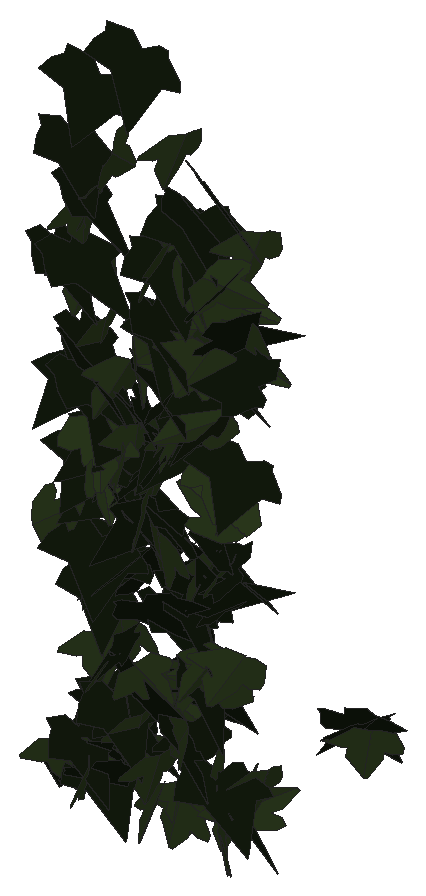
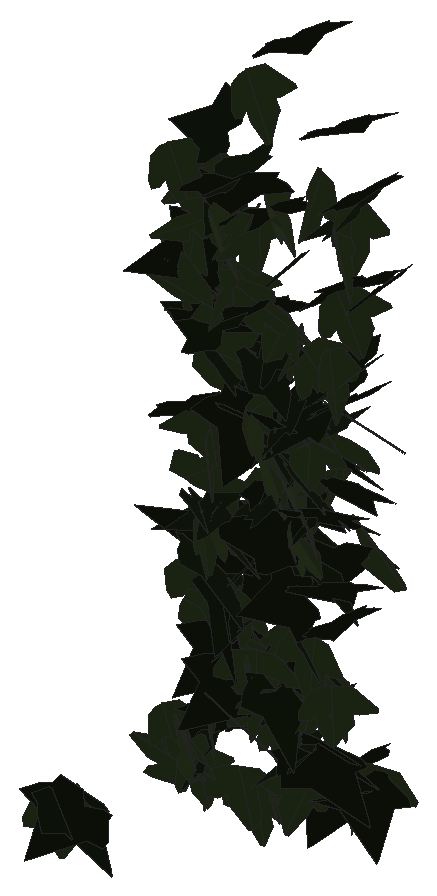
# SketchUp Ruby script. Lengths in inches.
U = 1.inch
M = Sketchup.active_model
def pt(a) = Geom::Point3d.new(a.map { |v| v * U })
def face(e, loops, mat)
  f = e.add_face(loops[0].map { |a| pt(a) })
  loops[1..].each { |l| e.add_face(l.map { |a| pt(a) }).erase! }
  f.material = f.back_material = mat if mat
  f
end
# faces: each face lists its corners as indices into pts; further lists are holes
def faces(e, pts, list, mat = nil) = list.each { |f| face(e, (f[0].is_a?(Array) ? f : [f]).map { |l| l.map { |i| pts[i] } }, mat) }
# xy, xz, yz: faces in a plane at the given z, y or x. An outline is a flat list of corners, or four numbers for a rectangle; further outlines are holes
def ring(l) = l.size == 4 ? [[l[0], l[1]], [l[2], l[1]], [l[2], l[3]], [l[0], l[3]]] : l.each_slice(2).to_a
def flat(e, list, mat, &to3) = list.each { |f| face(e, (f[0].is_a?(Array) ? f : [f]).map { |l| ring(l).map { |u, v| to3.(u, v) } }, mat) }
def xy(e, z, list, mat = nil) = flat(e, list, mat) { |x, y| [x, y, z] }
def xz(e, y, list, mat = nil) = flat(e, list, mat) { |x, z| [x, y, z] }
def yz(e, x, list, mat = nil) = flat(e, list, mat) { |y, z| [x, y, z] }
def lines(e, pts, list) = list.each { |a, b| e.add_line(pt(pts[a]), pt(pts[b])) }
# prism: a flat outline (further loops are holes) pulled along v
def prism(e, loops, v, mat = nil)
  f = face(e, loops, mat); d = Geom::Vector3d.new(v.map { |x| x * U })
  f.pushpull(f.normal.samedirection?(d) ? d.length : -d.length)
end
def box(e, o, s, mat = nil) = prism(e, [[o, [o[0] + s[0], o[1], o[2]], [o[0] + s[0], o[1] + s[1], o[2]], [o[0], o[1] + s[1], o[2]]]], [0, 0, s[2]], mat)
def at(x, y, z, deg = 0) = Geom::Transformation.translation(pt([x, y, z])) * Geom::Transformation.rotation(ORIGIN, Z_AXIS, deg.degrees)
def axes(o, x, y, z) = Geom::Transformation.new([*x, 0, *y, 0, *z, 0, *pt(o).to_a, 1])
def part(name) = M.definitions.add(name)
# library, detail: a bought-in or finely detailed component or shape, given as its bounding box
def library(name, o, s) = part(name).tap { |d| box(d.entities, o, s) }
def detail(e, o, s) = box(e.add_group.entities, o, s)
def put(e, d, t, mat = nil) = e.add_instance(d, t).tap { |i| i.material = mat if mat }
def group(e, t, mat = nil) = e.add_group.tap { |g| g.transformation = t; g.material = mat if mat }.entities
root = M.entities
M.materials.add("1026 AP 7946 SUNNY SIDE UP").color = [254, 231, 186]
M.materials.add("efeu1").color = [18, 25, 13]
M.materials.add("efeu2").color = [43, 57, 29]
c1 = part("ivyleaf_10")
p = [[0,0.5,-0.03],[-0.0625,2.02,-0.43],[-0.19,2.01,-0.46],[-0.54,1.05,-0.29],[-0.52,0.625,-0.18],[-0.83,0.76,-0.28],
  [-1.16,0.64,-0.33],[-1.15,0.33,-0.24],[-0.77,-0.39,0.02],[-0.3,-0.51,0.16],[0.04,-0.48,0.23],[-0.02,2.01,-0.4375],
  [-0.06,2.01,-0.43],[0.04,-0.49,0.23],[0.67,-0.49,0.14],[1.38,0.36,-0.2],[1.375,0.51,-0.24],[0.81,0.65,-0.19],
  [0.62,0.59,-0.15],[0.6,1.09,-0.28],[0.5,1.23,-0.31]]
faces(c1.entities,p,[[0,1,2,3,4,5,6,7,8,9,10],[11,12,0,13,14,15,16,17,18,19,20]],"efeu2")
c2 = part("ivyleaf_9")
p = [[1.54,2.16,1.25],[1.36,2.04,1.19],[-0.21,0.99,0.68],[-0.71,1.11,0.82],[-0.85,0.86,0.67],[-0.8,0.17,0.21],
  [-0.9,-0.01,0.1],[-0.67,-0.16,-0.02],[-0.08,-0.08,-0.05],[-0.03,-0.6,-0.4],[0.65,-0.88,-0.66],[0.83,-0.6,-0.49],
  [1.29,-0.42,-0.43],[1.8125,-0.07,-0.26],[1.21,0.44,0.15]]
faces(c2.entities,p,[[0,1,2,3,4,5,6,7,8,9,10,11,12,13,14]],"efeu1")
put(root,c1,axes([128.77,212.34,283.15],[0.31487,-0.18449,-0.22671],[0.28999,-0.12137,0.27832],[-0.34447,-0.27081,0.02707]),"1026 AP 7946 SUNNY SIDE UP")
put(root,c2,axes([128.875,212.4,287.29],[0.16277,-0.31766,-0.09668],[-0.03791,0.08894,-0.34364],[0.51865,0.10619,0.00522]),"1026 AP 7946 SUNNY SIDE UP")
put(root,c2,axes([129.22,212.62,285.39],[-0.49049,-0.04517,-0.10193],[0.16934,-0.09172,-0.30799],[0.02108,-0.31405,0.10257]),"1026 AP 7946 SUNNY SIDE UP")
put(root,c2,axes([128.96,212.68,288.75],[-0.00054,-0.35085,-0.02221],[0.01961,0.01954,-0.3611],[0.55219,-0.00104,0.0128]),"1026 AP 7946 SUNNY SIDE UP")
put(root,c2,axes([129.28,212.29,279.97],[0.19093,0.26653,-0.14134],[-0.09154,-0.12591,-0.30246],[-0.4635,0.13466,0.00151]),"1026 AP 7946 SUNNY SIDE UP")
put(root,c1,axes([129.2,212.18,280],[-0.40377,-0.18367,-0.07564],[0.11643,0.02048,-0.32404],[0.28776,-0.266,0.02498]),"1026 AP 7946 SUNNY SIDE UP")
put(root,c1,axes([129.27,212.73,287.93],[0.13295,-0.33199,-0.07426],[-0.00651,0.07133,-0.35224],[0.53352,0.0836,0.01421]),"1026 AP 7946 SUNNY SIDE UP")
put(root,c1,axes([129.3,212.62,286.95],[-0.20815,-0.31172,0.08991],[0.00262,-0.09684,-0.34724],[0.50974,-0.12679,0.0385]),"1026 AP 7946 SUNNY SIDE UP")
put(root,c2,axes([129.25,212.82,289.65],[-0.24116,-0.30442,0.09077],[0.00826,-0.10219,-0.34812],[0.49901,-0.14543,0.04962]),"1026 AP 7946 SUNNY SIDE UP")
put(root,c1,axes([129.36,212.79,281.35],[-0.30602,-0.25261,0.0146],[0.0642,-0.05076,-0.32229],[0.39275,-0.18853,0.06405]),"1026 AP 7946 SUNNY SIDE UP")
put(root,c1,axes([129.37,212.35,288.04],[-0.0998,-0.33764,-0.07705],[0.04363,0.06887,-0.35322],[0.54138,-0.06779,0.01426]),"1026 AP 7946 SUNNY SIDE UP")
put(root,c1,axes([129.4,212.71,286.11],[-0.02529,-0.33428,-0.08226],[0.01042,0.07772,-0.3443],[0.53962,-0.01717,0.00279]),"1026 AP 7946 SUNNY SIDE UP")
put(root,c2,axes([129.13,212.65,286.02],[0.19765,-0.30445,-0.09302],[-0.01495,0.09161,-0.33779],[0.49833,0.1235,0.02676]),"1026 AP 7946 SUNNY SIDE UP")
put(root,c2,axes([129.6,212.85,280.47],[0.14491,0.11175,-0.28967],[-0.24026,-0.23728,-0.14979],[-0.41172,0.1778,-0.01454]),"1026 AP 7946 SUNNY SIDE UP")
put(root,c2,axes([129.16,212.41,287.3],[0.12708,-0.29012,-0.17529],[0.07618,0.1816,-0.29711],[0.52202,0.04413,0.08603]),"1026 AP 7946 SUNNY SIDE UP")
put(root,c2,axes([129.54,212.59,284.34],[-0.46172,-0.14613,-0.05063],[0.11028,-0.0344,-0.33213],[0.21543,-0.29559,0.06151]),"1026 AP 7946 SUNNY SIDE UP")
put(root,c2,axes([129.24,212.43,288.28],[0.27121,-0.30689,-0.07246],[-0.0126,0.07392,-0.36103],[0.49431,0.17027,0.03055]),"1026 AP 7946 SUNNY SIDE UP")
put(root,c2,axes([129.36,212.3,280.26],[0.04395,-0.30745,-0.10444],[-0.01885,0.09895,-0.31744],[0.50783,0.03028,-0.00274]),"1026 AP 7946 SUNNY SIDE UP")
put(root,c1,axes([129.55,212.77,288.64],[-0.00548,-0.23836,-0.29542],[0.05999,0.28368,-0.2429],[0.58161,-0.03151,0.02227]),"1026 AP 7946 SUNNY SIDE UP")
put(root,c2,axes([129.4375,212.67,282.38],[-0.09606,-0.32529,0.02138],[-0.00287,-0.02265,-0.3411],[0.51272,-0.06107,0.0021]),"1026 AP 7946 SUNNY SIDE UP")
put(root,c2,axes([129.77,212.75,280.62],[-0.50354,0.00349,-0.01504],[0.02207,-0.04213,-0.32733],[-0.00845,-0.31779,0.04134]),"1026 AP 7946 SUNNY SIDE UP")
put(root,c2,axes([129.29,212.41,285.57],[0.19261,-0.28911,-0.16675],[0.0311,0.17697,-0.31237],[0.5188,0.09673,0.08063]),"1026 AP 7946 SUNNY SIDE UP")
put(root,c1,axes([129.61,212.09,279.8125],[0.10943,-0.27423,-0.15568],[-0.01177,0.15172,-0.28929],[0.49101,0.06475,0.02776]),"1026 AP 7946 SUNNY SIDE UP")
put(root,c2,axes([129.58,212.78,282.88],[-0.32897,-0.25226,0.02968],[0.03288,-0.05614,-0.33372],[0.39814,-0.2038,0.05209]),"1026 AP 7946 SUNNY SIDE UP")
put(root,c2,axes([129.31,212.26,285.95],[0.32591,-0.26952,0.0464],[0.01664,-0.05049,-0.34982],[0.42975,0.20635,-0.02164]),"1026 AP 7946 SUNNY SIDE UP")
put(root,c1,axes([129.65,212.46,281.25],[0.11967,-0.31363,-0.0036],[-0.01012,0.0002,-0.33242],[0.49306,0.07612,-0.00595]),"1026 AP 7946 SUNNY SIDE UP")
put(root,c2,axes([129.8,212.78,283.88],[-0.46379,-0.1306,0.08783],[-0.06846,-0.10776,-0.32304],[0.23616,-0.28772,0.07885]),"1026 AP 7946 SUNNY SIDE UP")
put(root,c1,axes([129.8,212.68,281.86],[-0.48011,0.0946,0.04933],[-0.08062,-0.00584,-0.32866],[-0.14549,-0.30893,0.01934]),"1026 AP 7946 SUNNY SIDE UP")
put(root,c2,axes([129.65,212.21,279.81],[0.32277,0.23557,-0.0003],[0.02221,-0.01446,-0.32131],[-0.36975,0.20477,-0.01956]),"1026 AP 7946 SUNNY SIDE UP")
put(root,c2,axes([129.91,212.51,284.73],[-0.52122,-0.00918,-0.03163],[0.05013,-0.06745,-0.33475],[0.0043,-0.32599,0.06817]),"1026 AP 7946 SUNNY SIDE UP")
put(root,c2,axes([129.55,212.52,279.73],[-0.06473,-0.30275,-0.08361],[0.09228,0.07124,-0.3106],[0.48343,-0.05413,0.04809]),"1026 AP 7946 SUNNY SIDE UP")
put(root,c1,axes([129.86,212.67,284.86],[-0.51512,0.04532,0.04355],[-0.07068,-0.01925,-0.33984],[-0.06667,-0.32972,0.02385]),"1026 AP 7946 SUNNY SIDE UP")
put(root,c2,axes([129.7,212.31,283.19],[-0.34121,-0.2423,-0.11903],[0.14727,0.06902,-0.33389],[0.39458,-0.23528,0.02168]),"1026 AP 7946 SUNNY SIDE UP")
put(root,c1,axes([129.63,212.31,284.76],[0.53185,-0.01594,0.1042],[0.15511,-0.04395,-0.34694],[0.04366,0.35032,-0.0367]),"1026 AP 7946 SUNNY SIDE UP")
put(root,c1,axes([129.74,212.3,284.23],[0.09294,0.32094,-0.02856],[0.00039,-0.03008,-0.33632],[-0.50679,0.05883,-0.0055]),"1026 AP 7946 SUNNY SIDE UP")
put(root,c1,axes([129.77,212.78,279.95],[0.23329,0.24155,0.15104],[-0.03258,0.17303,-0.27365],[-0.44198,0.11474,0.09989]),"1026 AP 7946 SUNNY SIDE UP")
put(root,c2,axes([129.74,212.53,284.91],[-0.16662,-0.25075,0.2084],[0.03989,-0.22019,-0.2669],[0.50642,-0.06516,0.08959]),"1026 AP 7946 SUNNY SIDE UP")
put(root,c2,axes([130.01,212.77,284.41],[-0.44334,0.11575,-0.13747],[0.16419,-0.09502,-0.31123],[-0.225,-0.29741,0.04375]),"1026 AP 7946 SUNNY SIDE UP")
put(root,c1,axes([130.01,212.36,285.8],[-0.09987,-0.30957,0.16238],[-0.00305,-0.16169,-0.32529],[0.54749,-0.05737,0.02781]),"1026 AP 7946 SUNNY SIDE UP")
put(root,c2,axes([129.76,212.55,285.33],[0.45438,-0.12423,-0.13502],[-0.16783,0.08034,-0.32217],[0.22805,0.30667,0.03192]),"1026 AP 7946 SUNNY SIDE UP")
put(root,c1,axes([129.95,212.69,283.9],[0.25028,-0.2959,0.01977],[0.01617,-0.01817,-0.34624],[0.46615,0.1595,0.0014]),"1026 AP 7946 SUNNY SIDE UP")
put(root,c2,axes([130.08,212.46,281.85],[-0.35019,0.16021,-0.17806],[0.19753,-0.12198,-0.28246],[-0.31479,-0.25477,0.02084]),"1026 AP 7946 SUNNY SIDE UP")
put(root,c1,axes([129.93,212.66,280.77],[-0.11128,0.30287,-0.07136],[0.00447,-0.07217,-0.32055],[-0.48912,-0.06957,0.0133]),"1026 AP 7946 SUNNY SIDE UP")
put(root,c2,axes([129.78,212.68,280.49],[0.31703,-0.21536,-0.13476],[-0.07859,0.12846,-0.29928],[0.38731,0.20234,0.04958]),"1026 AP 7946 SUNNY SIDE UP")
put(root,c1,axes([130.02,212.64,283.39],[0.10629,-0.29952,0.14076],[0.04339,-0.13558,-0.31711],[0.51696,0.07296,-0.00233]),"1026 AP 7946 SUNNY SIDE UP")
put(root,c2,axes([130.24,212.16,283.04],[-0.21219,0.30412,-0.08457],[0.02603,-0.08421,-0.34273],[-0.49535,-0.1347,0.01821]),"1026 AP 7946 SUNNY SIDE UP")
put(root,c2,axes([129.93,212.67,282.57],[0.14675,0.14689,0.32705],[0.26969,0.26615,-0.17773],[-0.478,0.19526,0.00013]),"1026 AP 7946 SUNNY SIDE UP")
put(root,c2,axes([130.2,212.88,281.2],[-0.02933,0.31867,-0.00245],[0.0019,-0.00412,-0.32888],[-0.50112,-0.01867,-0.0011]),"1026 AP 7946 SUNNY SIDE UP")
put(root,c1,axes([130.12,212.15,284.66],[0.23511,-0.26633,-0.15181],[-0.06004,0.14479,-0.31186],[0.47367,0.15055,0.03583]),"1026 AP 7946 SUNNY SIDE UP")
put(root,c2,axes([129.96,212.32,280.9375],[-0.02087,-0.32728,-0.09806],[0.01665,0.09296,-0.33683],[0.53488,-0.01566,0.00666]),"1026 AP 7946 SUNNY SIDE UP")
put(root,c2,axes([129.88,212.54,283.78],[0.32254,-0.26446,0.04331],[0.0179,-0.04619,-0.3445],[0.42106,0.20454,-0.01853]),"1026 AP 7946 SUNNY SIDE UP")
put(root,c2,axes([130.1,212.59,285.26],[0.35413,-0.14226,-0.20943],[-0.24688,0.12948,-0.27286],[0.30077,0.27378,0.02262]),"1026 AP 7946 SUNNY SIDE UP")
put(root,c1,axes([130.15,212.52,286.04],[-0.11065,0.30914,-0.10331],[0.00549,-0.10367,-0.32666],[-0.51186,-0.06794,0.01883]),"1026 AP 7946 SUNNY SIDE UP")
put(root,c1,axes([130.26,212.37,280.67],[-0.10037,-0.32889,-0.02865],[0.00829,0.0254,-0.34499],[0.51869,-0.06405,-0.00003]),"1026 AP 7946 SUNNY SIDE UP")
put(root,c1,axes([130.25,212.34,284.97],[-0.16104,-0.3145,-0.00569],[0.03661,-0.00366,-0.33992],[0.4932,-0.10242,0.02338]),"1026 AP 7946 SUNNY SIDE UP")
put(root,c2,axes([130.18,212.53,290.48],[-0.17086,-0.34818,0.04872],[-0.01103,-0.04942,-0.37595],[0.55282,-0.10859,0.00756]),"1026 AP 7946 SUNNY SIDE UP")
put(root,c2,axes([130.49,212.51,284.59],[-0.34855,0.19164,-0.15819],[0.1519,-0.12371,-0.30132],[-0.35617,-0.2403,0.0263]),"1026 AP 7946 SUNNY SIDE UP")
put(root,c1,axes([130.3,212.64,286.36],[-0.41948,0.1825,-0.08744],[0.0693,-0.08628,-0.33028],[-0.30951,-0.26666,0.04457]),"1026 AP 7946 SUNNY SIDE UP")
put(root,c1,axes([130.31,212.86,281.08],[0.01598,0.31311,0.06602],[-0.00803,0.06249,-0.32228],[-0.50192,0.00897,0.00726]),"1026 AP 7946 SUNNY SIDE UP")
put(root,c1,axes([130.43,212.7,284.33],[0.07673,-0.33132,-0.00821],[-0.01555,0.0047,-0.34485],[0.52082,0.04895,-0.00908]),"1026 AP 7946 SUNNY SIDE UP")
put(root,c1,axes([130.79,212.66,286.55],[-0.18229,0.07633,0.31542],[-0.49356,-0.05678,-0.10835],[0.04381,-0.32201,0.09182]),"1026 AP 7946 SUNNY SIDE UP")
put(root,c2,axes([130.56,212.36,283.85],[0.00799,0.09235,-0.33297],[0.01354,-0.32371,-0.09688],[-0.52918,-0.00689,-0.0075]),"1026 AP 7946 SUNNY SIDE UP")
put(root,c1,axes([130.29,212.72,281.05],[-0.3245,-0.12843,-0.21433],[0.30427,0.07905,-0.24843],[0.23338,-0.28164,0.02588]),"1026 AP 7946 SUNNY SIDE UP")
put(root,c1,axes([130.35,212.43,283.98],[0.21595,-0.21092,0.23039],[0.17894,-0.19407,-0.2603],[0.45051,0.17819,-0.00705]),"1026 AP 7946 SUNNY SIDE UP")
put(root,c1,axes([130.44,212.52,279.6],[0.07535,-0.28059,0.14542],[0.08514,-0.1349,-0.29267],[0.48764,0.06691,0.02863]),"1026 AP 7946 SUNNY SIDE UP")
put(root,c1,axes([130.52,212.77,284.88],[0.03751,-0.32466,0.07211],[0.0158,-0.07129,-0.33574],[0.5226,0.02546,0.00498]),"1026 AP 7946 SUNNY SIDE UP")
put(root,c2,axes([130.17,212.375,281.2],[0.13335,-0.11257,0.30199],[0.24026,-0.25123,-0.14608],[0.43242,0.1743,-0.01196]),"1026 AP 7946 SUNNY SIDE UP")
put(root,c2,axes([130.75,212.48,285.5625],[-0.21965,0.30146,-0.05079],[0.01903,-0.05059,-0.34241],[-0.48037,-0.13984,0.00966]),"1026 AP 7946 SUNNY SIDE UP")
put(root,c2,axes([130.1,212.8,283.36],[0.35825,-0.12911,0.20589],[0.28806,-0.08296,-0.26986],[0.24025,0.292,0.01655]),"1026 AP 7946 SUNNY SIDE UP")
put(root,c1,axes([130.64,212.74,281.39],[-0.48029,-0.10484,0.02286],[-0.01607,-0.04,-0.33103],[0.16793,-0.30368,0.03369]),"1026 AP 7946 SUNNY SIDE UP")
put(root,c1,axes([130.49,212.15,281.59],[-0.18567,-0.23753,-0.18173],[0.20174,0.12846,-0.26798],[0.41781,-0.16759,0.04863]),"1026 AP 7946 SUNNY SIDE UP")
put(root,c1,axes([130.59,212.87,281.3],[0.24037,-0.28108,0.01464],[0.03948,-0.0043,-0.329],[0.4409,0.15362,0.02147]),"1026 AP 7946 SUNNY SIDE UP")
put(root,c1,axes([130.75,212.66,279.44],[-0.45491,0.08873,0.07807],[-0.14436,-0.05011,-0.30293],[-0.11241,-0.29472,0.07308]),"1026 AP 7946 SUNNY SIDE UP")
put(root,c2,axes([130.35,212.64,283.88],[0.28341,-0.27656,-0.01678],[-0.00792,0.01428,-0.33997],[0.43541,0.18027,0.00474]),"1026 AP 7946 SUNNY SIDE UP")
put(root,c2,axes([130.73,212.77,284.94],[-0.48787,-0.11451,-0.05786],[0.10902,-0.02943,-0.33683],[0.16779,-0.31382,0.0506]),"1026 AP 7946 SUNNY SIDE UP")
put(root,c2,axes([130.4,212.73,282.34],[0.21142,-0.29125,-0.06341],[-0.01822,0.06055,-0.32978],[0.46719,0.13417,0.01583]),"1026 AP 7946 SUNNY SIDE UP")
put(root,c1,axes([130.7,212.2,280.3],[-0.11195,-0.32635,-0.00173],[0.00728,-0.00119,-0.34408],[0.51309,-0.07119,0.00451]),"1026 AP 7946 SUNNY SIDE UP")
put(root,c1,axes([130.6,212.74,287.58],[0.14962,0.34033,-0.08836],[-0.0313,-0.0855,-0.36453],[-0.55174,0.09714,-0.00328]),"1026 AP 7946 SUNNY SIDE UP")
put(root,c1,axes([130.65,212.74,284.93],[0.03949,-0.28865,0.17004],[0.09059,-0.16089,-0.2969],[0.51624,0.05032,0.03909]),"1026 AP 7946 SUNNY SIDE UP")
put(root,c1,axes([130.7,212.29,287.78],[0.17533,-0.32492,0.06543],[0.01039,-0.06676,-0.35393],[0.52103,0.11067,-0.01496]),"1026 AP 7946 SUNNY SIDE UP")
put(root,c2,axes([130.42,212.6,285.67],[0.05264,-0.26682,0.21707],[0.14708,-0.19788,-0.27265],[0.51551,0.0837,0.05562]),"1026 AP 7946 SUNNY SIDE UP")
put(root,c2,axes([130.68,212.73,286.5],[-0.25428,-0.30142,-0.00255],[0.01506,-0.00427,-0.35225],[0.47372,-0.16166,0.00983]),"1026 AP 7946 SUNNY SIDE UP")
put(root,c2,axes([130.53,212.37,286.86],[0.15621,-0.32994,-0.0227],[-0.01478,0.01822,-0.35485],[0.51955,0.09972,-0.00327]),"1026 AP 7946 SUNNY SIDE UP")
put(root,c1,axes([130.83,212.18,283.61],[-0.42763,0.19552,0.05338],[-0.09292,0.00429,-0.34358],[-0.3037,-0.27661,0.02997]),"1026 AP 7946 SUNNY SIDE UP")
put(root,c2,axes([130.64,212.0625,282.68],[0.39587,0.21816,0.02149],[0.04969,-0.0066,-0.34221],[-0.34081,0.25244,-0.02494]),"1026 AP 7946 SUNNY SIDE UP")
put(root,c2,axes([130.7,212.6,284.89],[0.39777,0.2194,-0.04297],[-0.01842,-0.05177,-0.34377],[-0.35104,0.25131,-0.03065]),"1026 AP 7946 SUNNY SIDE UP")
put(root,c1,axes([130.91,212.7,279.62],[-0.44589,-0.10915,0.07147],[-0.07841,-0.06357,-0.31063],[0.1882,-0.28508,0.0399]),"1026 AP 7946 SUNNY SIDE UP")
put(root,c1,axes([130.9375,212.4,289.46],[-0.1248,-0.35289,0.03585],[-0.00867,-0.03648,-0.37283],[0.55782,-0.07952,0.00222]),"1026 AP 7946 SUNNY SIDE UP")
put(root,c2,axes([131.17,212.87,280.73],[-0.43758,0.15369,-0.00252],[-0.01542,-0.02461,-0.32653],[-0.24123,-0.27722,0.02545]),"1026 AP 7946 SUNNY SIDE UP")
put(root,c1,axes([131.21,212.45,286.33],[0.29242,-0.03514,-0.29071],[-0.44079,0.03253,-0.19444],[0.0732,0.33622,-0.00956]),"1026 AP 7946 SUNNY SIDE UP")
put(root,c2,axes([130.76,212.39,287.73],[-0.0905,-0.33695,-0.07653],[0.05095,0.06776,-0.35115],[0.5395,-0.06292,0.02033]),"1026 AP 7946 SUNNY SIDE UP")
put(root,c1,axes([130.85,212.76,282.24],[0.4374,-0.17127,0.03048],[0.08894,0.03453,-0.33084],[0.2587,0.27771,0.06221]),"1026 AP 7946 SUNNY SIDE UP")
put(root,c2,axes([130.76,212.79,281.1],[0.43002,0.15676,0.06922],[0.09976,0.02255,-0.32438],[-0.24834,0.2805,-0.01044]),"1026 AP 7946 SUNNY SIDE UP")
put(root,c2,axes([131.23,212.73,281.95],[0.03863,0.04669,-0.33168],[-0.48878,0.09949,-0.00898],[0.1523,0.30747,0.0553]),"1026 AP 7946 SUNNY SIDE UP")
put(root,c1,axes([130.98,212.45,287.58],[-0.04433,0.32379,0.10371],[-0.03079,0.09745,-0.33408],[-0.53142,-0.03266,0.0107]),"1026 AP 7946 SUNNY SIDE UP")
put(root,c2,axes([131.13,212.64,282.14],[0.04988,0.27174,0.18648],[0.04731,0.1771,-0.28069],[-0.50987,0.04302,-0.0078]),"1026 AP 7946 SUNNY SIDE UP")
put(root,c2,axes([130.8125,212.52,280.67],[0.15191,-0.28859,0.13326],[0.04953,-0.12753,-0.3141],[0.49587,0.10114,-0.00945]),"1026 AP 7946 SUNNY SIDE UP")
put(root,c1,axes([131.15,212.51,286.45],[0.00031,0.07408,0.33909],[-0.17347,0.31063,-0.07023],[-0.50066,-0.10758,0.02454]),"1026 AP 7946 SUNNY SIDE UP")
put(root,c2,axes([130.89,212.61,282.62],[0.11468,-0.31558,0.0507],[-0.00034,-0.05236,-0.33376],[0.50265,0.07196,-0.01179]),"1026 AP 7946 SUNNY SIDE UP")
put(root,c2,axes([130.99,212.74,288.23],[-0.22022,-0.31537,-0.12785],[0.09481,0.10699,-0.35469],[0.52337,-0.15208,0.01045]),"1026 AP 7946 SUNNY SIDE UP")
put(root,c1,axes([131.2,212.1,280.97],[0.23814,-0.22842,-0.16716],[-0.08703,0.15493,-0.27925],[0.43068,0.15761,0.036]),"1026 AP 7946 SUNNY SIDE UP")
put(root,c1,axes([131.18,212.71,283.21],[0.05331,-0.28042,0.17778],[0.05467,-0.17107,-0.29173],[0.51616,0.04708,0.01254]),"1026 AP 7946 SUNNY SIDE UP")
put(root,c1,axes([131.43,212.51,285.48],[-0.17719,-0.1163,0.30894],[-0.2396,-0.26132,-0.16456],[0.4465,-0.18638,0.0343]),"1026 AP 7946 SUNNY SIDE UP")
put(root,c2,axes([130.93,212.67,288.29],[0.0555,-0.31784,0.15039],[0.0973,-0.14055,-0.32745],[0.5425,0.05772,0.04334]),"1026 AP 7946 SUNNY SIDE UP")
put(root,c2,axes([131.46,212.64,282.62],[-0.07659,0.31556,0.07411],[-0.11358,0.05852,-0.32253],[-0.49545,-0.0622,0.06248]),"1026 AP 7946 SUNNY SIDE UP")
put(root,c2,axes([131,212.66,281.44],[0.4965,0.06116,0.0054],[0.01808,-0.03376,-0.32953],[-0.09477,0.31399,-0.03455]),"1026 AP 7946 SUNNY SIDE UP")
put(root,c1,axes([131.25,212.72,287.5],[0.16903,-0.33066,0.03095],[0.00327,-0.03288,-0.35829],[0.52234,0.10721,-0.00777]),"1026 AP 7946 SUNNY SIDE UP")
put(root,c1,axes([131.4,212.35,286.49],[-0.37265,-0.19093,0.14873],[-0.11388,-0.138,-0.30899],[0.35983,-0.24141,0.05624]),"1026 AP 7946 SUNNY SIDE UP")
put(root,c1,axes([131.22,212.48,287.32],[-0.13611,0.32593,-0.01968],[-0.01179,-0.02365,-0.34728],[-0.51341,-0.08587,0.01319]),"1026 AP 7946 SUNNY SIDE UP")
put(root,c1,axes([131.48,212.79,283.84],[0.25389,0.19689,0.22159],[-0.25199,-0.14396,0.26021],[0.3815,-0.22612,0.02441]),"1026 AP 7946 SUNNY SIDE UP")
put(root,c2,axes([131.1,212.66,281.48],[0.09187,-0.31032,0.06327],[0.00502,-0.06366,-0.32556],[0.49793,0.0579,-0.00839]),"1026 AP 7946 SUNNY SIDE UP")
put(root,c1,axes([131.69,212.54,281.71],[-0.16375,0.02232,0.32642],[-0.47549,-0.10858,-0.09518],[0.15219,-0.31523,0.05382]),"1026 AP 7946 SUNNY SIDE UP")
put(root,c2,axes([131.44,212.65,285.63],[-0.40539,0.12791,-0.1861],[0.21402,-0.12846,-0.2934],[-0.27565,-0.28786,0.04589]),"1026 AP 7946 SUNNY SIDE UP")
put(root,c1,axes([131.4,212.49,281.96],[-0.07173,-0.2424,0.21879],[-0.00623,-0.21544,-0.25382],[0.50814,-0.03686,0.02777]),"1026 AP 7946 SUNNY SIDE UP")
put(root,c1,axes([131.41,212.6875,284.28],[0.19724,-0.26768,-0.16854],[-0.02901,0.16799,-0.29954],[0.4912,0.11741,0.04998]),"1026 AP 7946 SUNNY SIDE UP")
put(root,c2,axes([131.57,212.73,286.125],[-0.47208,-0.14275,0.09049],[-0.11003,-0.05882,-0.34205],[0.24022,-0.30747,0.02117]),"1026 AP 7946 SUNNY SIDE UP")
put(root,c1,axes([131.4,212.81,283.13],[0.03187,-0.32068,-0.06284],[0.01617,0.05989,-0.33037],[0.5125,0.01805,0.01433]),"1026 AP 7946 SUNNY SIDE UP")
put(root,c2,axes([131.66,212.63,283.3],[-0.36123,0.23166,-0.01943],[-0.00303,-0.03025,-0.33547],[-0.36563,-0.22862,0.02197]),"1026 AP 7946 SUNNY SIDE UP")
put(root,c1,axes([131.36,212.73,284.62],[0.41756,0.2101,-0.02433],[-0.03093,-0.01513,-0.34893],[-0.33121,0.26628,0.00191]),"1026 AP 7946 SUNNY SIDE UP")
put(root,c2,axes([131.13,212.76,283.47],[0.3627,-0.23952,-0.01679],[0.04538,0.04826,-0.3377],[0.37461,0.22605,0.05717]),"1026 AP 7946 SUNNY SIDE UP")
put(root,c2,axes([131.03,212.46,282.79],[0.14919,0.00592,0.3546],[0.54123,-0.00551,-0.09769],[0.00588,0.35697,-0.0053]),"1026 AP 7946 SUNNY SIDE UP")
put(root,c1,axes([131.35,212.71,280.3],[0.14827,-0.2557,0.17114],[0.22232,-0.11902,-0.26974],[0.42622,0.15103,0.08116]),"1026 AP 7946 SUNNY SIDE UP")
put(root,c2,axes([131.13,212.84,286.08],[0.19518,-0.25905,0.18504],[0.20714,-0.13445,-0.29195],[0.45177,0.17356,0.05392]),"1026 AP 7946 SUNNY SIDE UP")
put(root,c1,axes([131.54,212.8,279.67],[-0.14165,-0.28207,0.0832],[0.03335,-0.09216,-0.3018],[0.46084,-0.08003,0.04741]),"1026 AP 7946 SUNNY SIDE UP")
put(root,c2,axes([131.23,212.6,288.8],[0.28901,-0.2573,0.16291],[0.11173,-0.14483,-0.3257],[0.4628,0.19565,-0.02311]),"1026 AP 7946 SUNNY SIDE UP")
put(root,c1,axes([131.61,212.76,279.88],[0.32824,-0.22962,0.03191],[0.02263,-0.03052,-0.31972],[0.36391,0.20902,-0.0089]),"1026 AP 7946 SUNNY SIDE UP")
put(root,c2,axes([131.73,211.94,287.5625],[0.09168,0.25417,0.2606],[0.04443,0.25076,-0.26635],[-0.5605,0.06145,0.02151]),"1026 AP 7946 SUNNY SIDE UP")
put(root,c1,axes([131.73,212.3,279.46],[-0.20893,0.25087,0.12643],[-0.1543,0.08365,-0.28847],[-0.41009,-0.15928,0.04413]),"1026 AP 7946 SUNNY SIDE UP")
put(root,c2,axes([131.84,215.02,280.01],[-0.08258,0.27854,-0.12618],[-0.04255,-0.12965,-0.28883],[-0.47757,-0.03661,0.04755]),"1026 AP 7946 SUNNY SIDE UP")
put(root,c1,axes([131.55,212.89,279.69],[0.18919,-0.28601,-0.03961],[0.03279,-0.03117,0.31939],[-0.45225,-0.12191,0.00659]),"1026 AP 7946 SUNNY SIDE UP")
put(root,c2,axes([131.69,212.78,284.8],[-0.27148,-0.28701,0.02843],[-0.00091,-0.03372,-0.34482],[0.45363,-0.17183,0.01632]),"1026 AP 7946 SUNNY SIDE UP")
put(root,c1,axes([131.78,212.65,287],[-0.43088,0.19407,0.04994],[-0.08885,0.00184,-0.34445],[-0.30129,-0.27809,0.03015]),"1026 AP 7946 SUNNY SIDE UP")
put(root,c2,axes([131.46,212.79,279.77],[0.28939,-0.25032,0.02074],[0.00173,-0.02592,-0.31989],[0.39506,0.18348,-0.01379]),"1026 AP 7946 SUNNY SIDE UP")
put(root,c2,axes([131.55,212.48,280.27],[-0.15126,-0.27248,-0.16854],[0.13803,0.13983,-0.29508],[0.479,-0.12634,0.03181]),"1026 AP 7946 SUNNY SIDE UP")
put(root,c2,axes([131.5625,215.07,280.02],[0.45256,0.11807,0.00277],[0.01917,-0.02442,-0.3194],[-0.18469,0.28679,-0.02636]),"1026 AP 7946 SUNNY SIDE UP")
put(root,c1,axes([131.48,212.38,287.39],[-0.14797,-0.15059,-0.32764],[0.42712,0.17685,-0.16849],[0.34983,-0.27962,0.06713]),"1026 AP 7946 SUNNY SIDE UP")
put(root,c1,axes([131.94,212.33,282.12],[-0.32985,-0.20266,0.15234],[-0.0866,-0.15233,-0.29417],[0.38594,-0.20738,0.06419]),"1026 AP 7946 SUNNY SIDE UP")
put(root,c1,axes([131.62,212.86,279.62],[-0.21675,-0.14663,0.24687],[0.22066,0.19637,0.20738],[-0.38397,0.19562,-0.02018]),"1026 AP 7946 SUNNY SIDE UP")
put(root,c2,axes([132.23,212.32,286.36],[-0.37331,0.20648,0.14555],[-0.24923,0.02458,-0.31386],[-0.30303,-0.27458,0.07883]),"1026 AP 7946 SUNNY SIDE UP")
put(root,c2,axes([131.61,212.31,286.8125],[0.27711,0.16144,0.28302],[0.3386,0.16965,-0.24484],[-0.36763,0.27794,-0.01217]),"1026 AP 7946 SUNNY SIDE UP")
put(root,c1,axes([131.9375,212.86,280.22],[-0.12246,-0.30496,0.02147],[-0.00267,-0.02287,-0.32436],[0.48082,-0.07779,0.00367]),"1026 AP 7946 SUNNY SIDE UP")
put(root,c1,axes([131.43,212.85,286.42],[0.03241,0.04065,0.38708],[0.59108,-0.03881,-0.01715],[0.0578,0.37406,-0.0416]),"1026 AP 7946 SUNNY SIDE UP")
put(root,c1,axes([131.97,215.03,279.86],[-0.36307,-0.2028,0.02567],[-0.00891,-0.03297,-0.31605],[0.32138,-0.23002,0.02024]),"1026 AP 7946 SUNNY SIDE UP")
put(root,c1,axes([131.95,212.71,288.21],[-0.20871,-0.31791,0.07182],[0.0133,-0.08056,-0.35321],[0.5122,-0.12745,0.03844]),"1026 AP 7946 SUNNY SIDE UP")
put(root,c1,axes([131.76,212.08,287.84],[-0.18403,-0.17969,-0.28713],[0.31481,0.19598,-0.21643],[0.41398,-0.22891,0.03695]),"1026 AP 7946 SUNNY SIDE UP")
